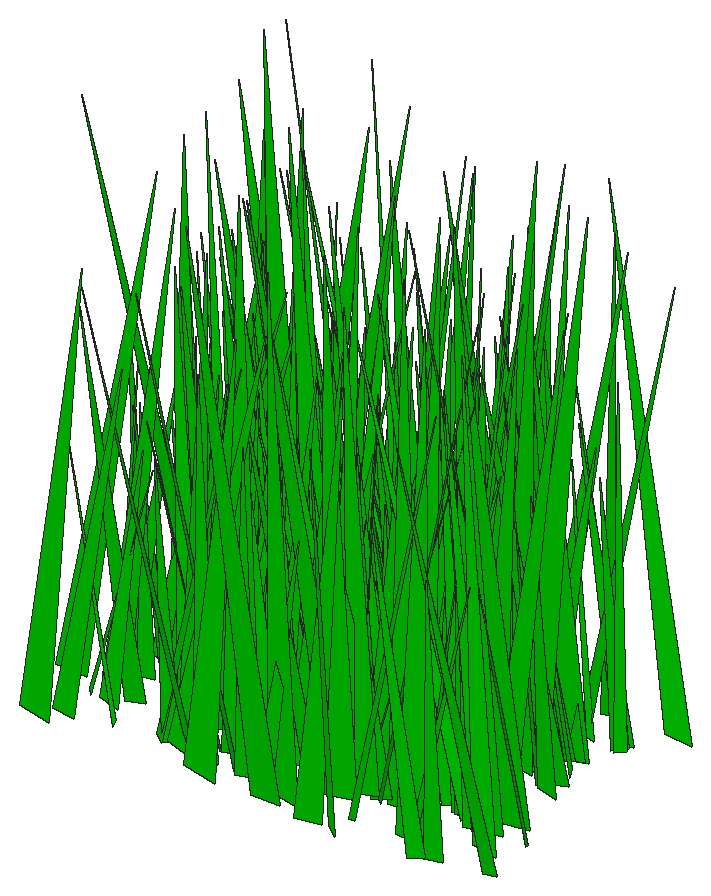
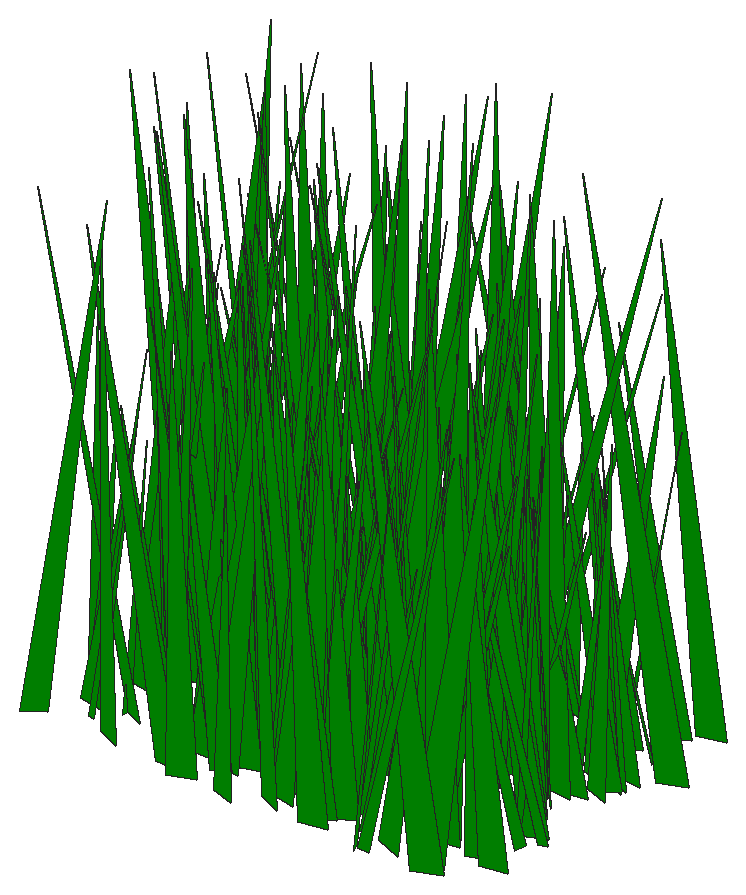
# SketchUp Ruby script. Lengths in inches.
U = 1.inch
M = Sketchup.active_model
def pt(a) = Geom::Point3d.new(a.map { |v| v * U })
def face(e, loops, mat)
  f = e.add_face(loops[0].map { |a| pt(a) })
  loops[1..].each { |l| e.add_face(l.map { |a| pt(a) }).erase! }
  f.material = f.back_material = mat if mat
  f
end
# faces: each face lists its corners as indices into pts; further lists are holes
def faces(e, pts, list, mat = nil) = list.each { |f| face(e, (f[0].is_a?(Array) ? f : [f]).map { |l| l.map { |i| pts[i] } }, mat) }
# xy, xz, yz: faces in a plane at the given z, y or x. An outline is a flat list of corners, or four numbers for a rectangle; further outlines are holes
def ring(l) = l.size == 4 ? [[l[0], l[1]], [l[2], l[1]], [l[2], l[3]], [l[0], l[3]]] : l.each_slice(2).to_a
def flat(e, list, mat, &to3) = list.each { |f| face(e, (f[0].is_a?(Array) ? f : [f]).map { |l| ring(l).map { |u, v| to3.(u, v) } }, mat) }
def xy(e, z, list, mat = nil) = flat(e, list, mat) { |x, y| [x, y, z] }
def xz(e, y, list, mat = nil) = flat(e, list, mat) { |x, z| [x, y, z] }
def yz(e, x, list, mat = nil) = flat(e, list, mat) { |y, z| [x, y, z] }
def lines(e, pts, list) = list.each { |a, b| e.add_line(pt(pts[a]), pt(pts[b])) }
# prism: a flat outline (further loops are holes) pulled along v
def prism(e, loops, v, mat = nil)
  f = face(e, loops, mat); d = Geom::Vector3d.new(v.map { |x| x * U })
  f.pushpull(f.normal.samedirection?(d) ? d.length : -d.length)
end
def box(e, o, s, mat = nil) = prism(e, [[o, [o[0] + s[0], o[1], o[2]], [o[0] + s[0], o[1] + s[1], o[2]], [o[0], o[1] + s[1], o[2]]]], [0, 0, s[2]], mat)
def at(x, y, z, deg = 0) = Geom::Transformation.translation(pt([x, y, z])) * Geom::Transformation.rotation(ORIGIN, Z_AXIS, deg.degrees)
def axes(o, x, y, z) = Geom::Transformation.new([*x, 0, *y, 0, *z, 0, *pt(o).to_a, 1])
def part(name) = M.definitions.add(name)
# library, detail: a bought-in or finely detailed component or shape, given as its bounding box
def library(name, o, s) = part(name).tap { |d| box(d.entities, o, s) }
def detail(e, o, s) = box(e.add_group.entities, o, s)
def put(e, d, t, mat = nil) = e.add_instance(d, t).tap { |i| i.material = mat if mat }
def group(e, t, mat = nil) = e.add_group.tap { |g| g.transformation = t; g.material = mat if mat }.entities
root = M.entities
M.materials.add("[Color G06]").color = [0, 204, 0]
c1 = part("fur_instance\#9")
p = [[0.8125,0,1.79],[0.67,-0.02,1.48],[0,-0.11,0],[0,0.11,0]]
faces(c1.entities,p,[[0,1,2,3]])
put(root,c1,axes([66.86,19.9375,4.28],[1.87865,0.36654,1.99521],[2.70408,-0.30217,0.68954],[-1.17442,-0.10942,4.77928]),"[Color G06]")
put(root,c1,axes([68.1,25.11,4.28],[-2.15525,0.67666,0.22206],[4.83152,0.29674,0.87415],[-0.4748,-0.05194,7.88732]),"[Color G06]")
put(root,c1,axes([67.18,22.58,4.28],[-3.47971,0.08197,1.69373],[0.53126,0.51017,-0.39823],[1.16085,0.01223,5.25931]),"[Color G06]")
put(root,c1,axes([66.52,24.42,4.28],[0.42309,0.57045,0.7628],[4.11466,-0.05401,-0.45808],[0.25485,-0.07503,6.12956]),"[Color G06]")
put(root,c1,axes([66.54,19.3,4.28],[3.07056,-0.08104,1.31793],[-0.44163,-0.44196,-0.8234],[-0.95931,-0.05592,4.59749]),"[Color G06]")
put(root,c1,axes([66.6875,19.39,4.28],[2.45678,0.23622,1.03552],[1.66363,-0.35564,0.50318],[-0.76296,-0.01482,4.43164]),"[Color G06]")
put(root,c1,axes([67.52,19.99,4.28],[-1.9205,-0.283,0.23807],[-1.99672,0.26782,0.59218],[0.39663,-0.02207,4.13384]),"[Color G06]")
put(root,c1,axes([66.43,15.94,4.28],[1.56121,0.60454,1.75227],[4.48997,-0.20626,-0.76122],[0.09967,-0.17771,6.84462]),"[Color G06]")
put(root,c1,axes([68.08,18.0625,4.28],[-1.81069,-0.46934,1.37248],[-3.48469,0.2363,-0.98663],[-0.16937,0.15593,5.62628]),"[Color G06]")
put(root,c1,axes([67.1,24.18,4.28],[-1.84112,0.58038,2.27158],[4.32564,0.28516,-0.53801],[0.96001,-0.17181,6.78063]),"[Color G06]")
put(root,c1,axes([65.73,18.35,4.28],[3.975,-0.58982,0.67635],[-4.2533,-0.55251,0.48784],[-0.07084,0.07718,8.66142]),"[Color G06]")
put(root,c1,axes([67.5,19.25,4.28],[0.83936,0.35374,1.12599],[2.5864,-0.13297,0.49205],[-0.5596,-0.08399,3.96306]),"[Color G06]")
put(root,c1,axes([66.66,19.55,4.28],[2.1428,-0.32761,1.15813],[-2.4734,-0.28656,0.91034],[-0.04931,0.13727,4.66448]),"[Color G06]")
put(root,c1,axes([68.16,24.67,4.28],[-2.63031,-0.31404,1.45688],[-2.40009,0.37075,-0.49867],[0.51157,0.12471,5.15122]),"[Color G06]")
put(root,c1,axes([68.36,16.83,4.28],[-3.11827,0.00052,0.78759],[0.08232,0.43605,0.69466],[0.52051,-0.06582,4.60843]),"[Color G06]")
put(root,c1,axes([67.36,21.62,4.28],[-1.40042,-0.37433,1.56996],[-2.74011,0.22344,0.66016],[0.89517,0.09832,4.47679]),"[Color G06]")
put(root,c1,axes([68.67,23.9,4.28],[-2.32217,-0.30899,0.40673],[-2.22908,0.31788,-0.68694],[-0.12359,0.07246,4.74777]),"[Color G06]")
put(root,c1,axes([67.42,21.06,4.28],[2.68454,-0.01038,1.27198],[0.07883,-0.38667,-0.73394],[-0.85066,-0.06857,3.94611]),"[Color G06]")
put(root,c1,axes([68.76,20.36,4.28],[-2.53339,0.15401,0.39707],[1.13348,0.3487,0.61732],[0.07498,-0.06768,4.08411]),"[Color G06]")
put(root,c1,axes([67.14,20.26,4.28],[1.41484,0.35356,0.45263],[2.55149,-0.19384,-0.42139],[0.10067,-0.05597,4.31898]),"[Color G06]")
put(root,c1,axes([66.32,22.73,4.28],[3.40849,0.26284,0.17789],[1.88535,-0.4715,-0.66404],[0.11163,-0.06222,5.7833]),"[Color G06]")
put(root,c1,axes([70,19.12,4.28],[-5.22641,-0.46331,0.41706],[-3.33362,0.72473,-0.82927],[-0.06343,0.08615,9.21882]),"[Color G06]")
put(root,c1,axes([66.74,22.54,4.28],[2.15826,-0.53872,0.51034],[-3.86774,-0.29494,0.77205],[0.28691,0.07652,6.56871]),"[Color G06]")
put(root,c1,axes([66.82,17.78,4.28],[2.69775,0.05613,0.15937],[0.4148,-0.37075,-0.68549],[-0.03623,-0.06547,4.01857]),"[Color G06]")
put(root,c1,axes([68.17,20.68,4.28],[0.33333,0.50099,1.6784],[3.73976,-0.06195,0.46517],[-0.42793,-0.15115,5.37257]),"[Color G06]")
put(root,c1,axes([67.84,20.44,4.28],[2.61459,-0.6557,1.97081],[-4.76436,-0.38828,-0.72114],[-1.07242,0.12639,8.00869]),"[Color G06]")
put(root,c1,axes([67.875,20.76,4.28],[3.06982,-0.09826,1.8059],[-0.52492,-0.45759,-0.86705],[-1.29654,-0.0474,4.62685]),"[Color G06]")
put(root,c1,axes([66.8,18.875,4.28],[4.09215,-0.51417,0.31047],[-3.65099,-0.56974,-0.89852],[-0.55613,-0.04305,8.18341]),"[Color G06]")
put(root,c1,axes([69.1875,23.38,4.28],[-3.00443,-0.33013,0.34527],[-2.37868,0.41728,-0.40146],[0.01445,0.04936,5.70282]),"[Color G06]")
put(root,c1,axes([68.5,22.24,4.28],[0.12511,0.4386,1.50938],[3.24988,-0.04162,0.78767],[-0.59262,-0.13566,4.63821]),"[Color G06]")
put(root,c1,axes([66.98,16.45,4.28],[2.6605,-0.3964,0.77865],[-2.88966,-0.36648,0.62248],[-0.04716,0.09278,5.7857]),"[Color G06]")
put(root,c1,axes([67.58,17.58,4.28],[0.01908,0.3952,0.29774],[2.79688,0.00227,-0.74606],[0.49908,-0.02781,4.16959]),"[Color G06]")
put(root,c1,axes([67.33,21.74,4.28],[2.2581,-0.40529,1.12701],[-2.99728,-0.31212,0.52087],[-0.17964,0.1131,5.47612]),"[Color G06]")
put(root,c1,axes([66.68,23.17,4.28],[3.54165,-0.16499,0.34756],[-1.2057,-0.48604,0.93878],[-0.018,0.09337,5.50131]),"[Color G06]")
put(root,c1,axes([69.64,25.65,4.28],[-4.18506,0.16157,0.59083],[1.18763,0.58346,0.46238],[0.29713,-0.05642,6.47367]),"[Color G06]")
put(root,c1,axes([67.75,21.26,4.28],[2.76117,0.06081,1.0314],[0.34689,-0.39465,0.59848],[-0.73896,0.04195,4.13483]),"[Color G06]")
put(root,c1,axes([69.21,25.2,4.28],[2.28754,0.39059,3.57758],[3.06302,-0.41996,0.89228],[-2.04786,-0.19184,5.3309]),"[Color G06]")
put(root,c1,axes([68.81,19.81,4.28],[0.33216,-0.36905,1.20751],[-2.69385,-0.06907,-0.76975],[-0.63266,0.10034,3.91151]),"[Color G06]")
put(root,c1,axes([68.78,23.68,4.28],[1.64627,-0.76449,2.9162],[-5.69845,-0.2691,-0.91794],[-1.17939,0.23306,8.50584]),"[Color G06]")
put(root,c1,axes([68.36,24.14,4.28],[-0.90357,-0.68837,2.42229],[-5.14418,0.15076,0.63516],[0.73005,0.2103,7.47357]),"[Color G06]")
put(root,c1,axes([69.47,21.03,4.28],[-3.7436,0.26959,1.66858],[2.08086,0.53147,0.56415],[0.80878,-0.11953,6.27184]),"[Color G06]")
put(root,c1,axes([69.19,20.0625,4.28],[0.16372,-0.57583,0.88536],[-4.12958,-0.03409,-0.84112],[-0.59134,0.07863,6.11904]),"[Color G06]")
put(root,c1,axes([69.25,20.49,4.28],[-4.87639,0.34442,2.38343],[2.40871,0.71498,-0.86054],[1.68574,-0.02531,8.12422]),"[Color G06]")
put(root,c1,axes([69.51,23.16,4.28],[0.01728,0.39517,1.39572],[2.89289,-0.03411,1.02939],[-0.7307,-0.1257,4.10846]),"[Color G06]")
put(root,c1,axes([67.69,25.59,4.28],[2.37057,-0.64778,0.92581],[-4.68012,-0.32216,0.87413],[0.24483,0.11379,7.74547]),"[Color G06]")
put(root,c1,axes([70.09,22.11,4.28],[-2.03665,-0.69248,0.21969],[-4.95861,0.28196,-0.58576],[-0.30712,0.03966,8.00048]),"[Color G06]")
put(root,c1,axes([69.45,20.67,4.28],[-0.23865,0.37319,1.09593],[2.74489,0.0167,0.68194],[-0.40691,-0.10623,3.95739]),"[Color G06]")
put(root,c1,axes([70.99,16.75,4.28],[-4.49676,-0.17942,0.26218],[-1.29851,0.62071,-0.95326],[-0.0085,0.09224,6.92513]),"[Color G06]")
put(root,c1,axes([68.88,21.76,4.28],[2.31214,0.17246,1.55813],[1.49477,-0.32472,-0.82607],[-0.61809,-0.14016,3.8309]),"[Color G06]")
put(root,c1,axes([69.52,23.7,4.28],[-1.56475,-0.35583,1.99839],[-2.84891,0.22263,-0.42902],[0.42773,0.18113,4.45309]),"[Color G06]")
put(root,c1,axes([69.87,25.6875,4.28],[-3.56069,0.01834,1.41738],[0.0277,0.51104,-0.60432],[0.95703,0.05346,5.29094]),"[Color G06]")
put(root,c1,axes([70.14,24.99,4.28],[-2.67002,0.12698,0.6552],[0.96677,0.37124,0.53513],[0.2946,-0.0674,4.18215]),"[Color G06]")
put(root,c1,axes([68.8,19.33,4.28],[2.11124,0.33037,1.52609],[2.57017,-0.28527,-0.84817],[-0.2233,-0.1599,4.6664]),"[Color G06]")
put(root,c1,axes([70.77,24.28,4.28],[-6.01659,-0.01708,1.91793],[-0.04628,0.85646,0.5517],[1.28826,-0.04899,8.97717]),"[Color G06]")
put(root,c1,axes([69.46,24.11,4.28],[3.88439,0.18749,2.22279],[1.24854,-0.58,0.74638],[-1.56873,0.00265,6.09796]),"[Color G06]")
put(root,c1,axes([70.89,20.8,4.28],[1.76802,-0.46536,3.87408],[-3.79882,-0.34664,-0.91072],[-1.85066,0.26697,5.57049]),"[Color G06]")
put(root,c1,axes([69.9375,22.14,4.28],[-2.30921,0.36852,1.8808],[2.72165,0.35258,-0.47168],[1.07715,-0.10084,5.22392]),"[Color G06]")
put(root,c1,axes([70.13,16.98,4.28],[1.25924,-0.38577,0.58888],[-2.69186,-0.18364,-0.96168],[-0.75007,0.01139,4.43995]),"[Color G06]")
put(root,c1,axes([69.6875,18.43,4.28],[2.63574,0.33516,0.9538],[2.34226,-0.37815,0.80643],[-0.83546,-0.00279,5.26991]),"[Color G06]")
put(root,c1,axes([70.56,17.34,4.28],[-2.39176,0.593,0.72625],[4.24328,0.33868,-0.55196],[0.56101,-0.03352,7.2711]),"[Color G06]")
put(root,c1,axes([71.41,17.43,4.28],[-3.23318,-0.07626,0.20624],[-0.5568,0.44941,-0.40903],[0.0899,0.04086,4.88376]),"[Color G06]")
put(root,c1,axes([70.07,22.83,4.28],[3.08996,-0.12092,1.88491],[-1.10884,-0.44997,0.74435],[-1.05497,0.11878,4.73848]),"[Color G06]")
put(root,c1,axes([71.2,22.44,4.28],[-1.9391,-0.26111,1.2844],[-2.05387,0.25798,-0.90149],[0.16274,0.14464,3.92666]),"[Color G06]")
put(root,c1,axes([72.3125,16.91,4.28],[-4.63411,-0.11914,0.54552],[-0.90008,0.63988,-1.0263],[0.23024,0.10358,6.96756]),"[Color G06]")
put(root,c1,axes([72.5625,23.87,4.28],[-5.03737,0.15992,0.47896],[1.16716,0.7016,0.50985],[0.23592,-0.05637,7.70452]),"[Color G06]")
put(root,c1,axes([70.64,17.21,4.28],[1.92034,0.64349,1.46988],[4.66024,-0.28183,0.57361],[-0.73787,-0.10529,7.44824]),"[Color G06]")
put(root,c1,axes([71.47,20.19,4.28],[-3.19334,0.26439,1.99081],[2.16495,0.45316,0.84359],[0.82592,-0.16563,5.48606]),"[Color G06]")
put(root,c1,axes([71.6,18.84,4.28],[-3.18635,0.38671,0.67327],[2.69516,0.44754,-1.0376],[0.79354,0.03276,6.22746]),"[Color G06]")
put(root,c1,axes([71.7,24.47,4.28],[2.18816,0.37389,2.89627],[2.82521,-0.37976,0.86384],[-1.72125,-0.14801,5.09981]),"[Color G06]")
put(root,c1,axes([70.85,24.09,4.28],[-0.32978,0.44304,1.07825],[3.23647,0.05616,-0.43984],[0.37426,-0.09529,4.75371]),"[Color G06]")
put(root,c1,axes([71.62,24.69,4.28],[-5.44694,0.14293,2.6999],[0.9286,0.8,-0.68034],[1.85785,0.01918,8.25575]),"[Color G06]")
put(root,c1,axes([70.64,18.29,4.28],[2.65428,-0.46035,0.81882],[-3.27632,-0.37734,-0.64678],[-0.68156,0.0211,6.29791]),"[Color G06]")
put(root,c1,axes([69.76,16.96,4.28],[4.07276,0.1691,0.72699],[1.2606,-0.56695,-0.62595],[-0.34363,-0.0756,6.32022]),"[Color G06]")
put(root,c1,axes([71.48,16.72,4.28],[0.89866,0.51945,1.33537],[3.77379,-0.14203,0.67396],[-0.6582,-0.10513,5.68738]),"[Color G06]")
put(root,c1,axes([70.92,24.74,4.28],[-2.03427,0.47242,2.51983],[3.53808,0.33213,-0.77265],[1.34233,-0.15948,5.85528]),"[Color G06]")
put(root,c1,axes([71.08,19.01,4.28],[-1.9152,0.36614,2.16956],[2.68071,0.31667,-0.85322],[1.34728,-0.10962,4.78176]),"[Color G06]")
put(root,c1,axes([71.48,19.53,4.28],[2.66418,0.13711,1.46624],[0.87126,-0.39543,0.71164],[-1.08175,0.01921,4.18426]),"[Color G06]")
put(root,c1,axes([71.09,18.5,4.28],[2.67934,-0.3919,0.38989],[-2.74937,-0.37373,-0.94945],[-0.63841,-0.03529,5.72518]),"[Color G06]")
put(root,c1,axes([70.22,23.08,4.28],[4.92283,0.46681,1.55066],[3.44128,-0.69107,-0.50511],[-0.66366,-0.12078,8.88315]),"[Color G06]")
put(root,c1,axes([71.08,18.49,4.28],[-0.01067,0.39008,0.75182],[2.75792,0.01838,-1.0079],[0.68705,-0.06771,4.05756]),"[Color G06]")
put(root,c1,axes([72.54,17.95,4.28],[-3.20854,0.5435,2.05319],[4.10111,0.44865,0.67282],[0.50943,-0.18866,7.51511]),"[Color G06]")
put(root,c1,axes([73.02,20.01,4.28],[-3.27762,0.0696,0.09378],[0.5027,0.45527,0.43295],[0.01818,-0.04125,4.93616]),"[Color G06]")
put(root,c1,axes([72.61,23.23,4.28],[-3.36746,-0.11854,0.93472],[-0.91893,0.47275,-0.50766],[0.51901,0.06791,5.16592]),"[Color G06]")
put(root,c1,axes([71.39,25.47,4.28],[0.0515,0.59852,1.18292],[4.35167,0.00142,-0.50587],[0.33469,-0.11059,6.39544]),"[Color G06]")
put(root,c1,axes([71.39,18.27,4.28],[0.1555,-0.38375,1.24845],[-2.85704,-0.00724,0.53918],[0.32964,0.11826,4.08421]),"[Color G06]")
put(root,c1,axes([70.56,16.81,4.28],[2.68875,0.54608,0.55936],[3.92681,-0.36876,-0.80773],[0.23645,-0.08553,7.05353]),"[Color G06]")
put(root,c1,axes([72.42,24.54,4.28],[2.08905,-0.57183,2.84194],[-4.26391,-0.34625,-1.00203],[-1.50031,0.18783,6.80495]),"[Color G06]")
put(root,c1,axes([71.76,19.93,4.28],[-2.5059,-0.08559,2.17745],[-0.46067,0.40376,0.63892],[1.51231,-0.01883,3.80266]),"[Color G06]")
put(root,c1,axes([71.65,22.36,4.28],[0.04403,-0.55707,0.45266],[-3.97735,-0.001,0.72254],[0.48148,0.04267,5.92718]),"[Color G06]")
put(root,c1,axes([71.96,17.59,4.28],[2.49858,-0.7621,1.22476],[-5.44507,-0.36092,-0.98619],[-0.94432,0.06469,8.92705]),"[Color G06]")
put(root,c1,axes([71.375,25.08,4.28],[2.08427,-0.50925,1.70734],[-3.82608,-0.27986,0.84419],[-0.05277,0.17755,6.22752]),"[Color G06]")
put(root,c1,axes([72.76,24.9375,4.28],[-0.44557,0.41686,0.30084],[2.96924,0.05764,0.64874],[-0.4009,-0.03642,4.47043]),"[Color G06]")
put(root,c1,axes([72.89,20,4.28],[2.34818,-0.68971,3.6819],[-5.24588,-0.39553,-1.038],[-1.73598,0.26228,8.11702]),"[Color G06]")
put(root,c1,axes([71.6,19.62,4.28],[1.93818,-0.4421,1.09106],[-3.25174,-0.26704,0.473],[-0.1042,0.11,5.53358]),"[Color G06]")
put(root,c1,axes([71.77,16.1,4.28],[0.44845,-0.59229,2.57221],[-4.55599,-0.03154,0.93997],[0.49558,0.24599,6.31381]),"[Color G06]")
put(root,c1,axes([72.95,19.9,4.28],[-4.47212,0.45643,2.42543],[3.3283,0.6565,-0.48377],[1.50651,-0.09547,8.26875]),"[Color G06]")
put(root,c1,axes([73.09,24.83,4.28],[-3.85958,0.09549,1.77507],[0.79917,0.55874,0.4286],[1.11393,-0.07,5.84281]),"[Color G06]")
put(root,c1,axes([74.125,22.51,4.28],[-4.09834,-0.08446,0.1041],[-0.59159,0.56687,0.80859],[0.14742,-0.07323,6.13878]),"[Color G06]")
put(root,c1,axes([72.22,20.39,4.28],[2.5598,0.08888,0.95436],[0.55163,-0.36615,0.61199],[-0.71391,0.03576,3.89483]),"[Color G06]")
put(root,c1,axes([72.79,16.75,4.28],[0.83062,0.44946,0.92704],[3.2366,-0.127,0.59543],[-0.5461,-0.06905,4.93894]),"[Color G06]")
put(root,c1,axes([74.5625,18.74,4.28],[-3.75514,0.60555,0.30301],[4.33004,0.51767,1.02411],[-0.38697,-0.08377,8.51899]),"[Color G06]")
put(root,c1,axes([72.64,23.35,4.28],[-1.03716,-0.47927,0.64226],[-3.42165,0.15149,0.64364],[0.53848,0.03948,5.3269]),"[Color G06]")
put(root,c1,axes([73.96,16.11,4.28],[-3.38072,-0.6515,1.18354],[-4.7345,0.47012,-0.48048],[0.20061,0.11585,8.60575]),"[Color G06]")
put(root,c1,axes([73.28,24.41,4.28],[0.14572,0.47172,1.353],[3.44856,-0.04129,0.82385],[-0.6085,-0.12101,4.99302]),"[Color G06]")
put(root,c1,axes([73.45,17.98,4.28],[-4.82019,0.18669,2.80146],[1.64531,0.70331,0.93941],[1.6121,-0.15958,7.4176]),"[Color G06]")
put(root,c1,axes([72.91,25.28,4.28],[3.98745,0.36913,2.2275],[2.62685,-0.59121,0.75083],[-1.52584,-0.05318,7.1137]),"[Color G06]")
put(root,c1,axes([74.33,17.61,4.28],[-2.66251,-0.38327,0.56727],[-2.77455,0.36742,-0.57227],[-0.0136,0.07516,5.6905]),"[Color G06]")
put(root,c1,axes([72.65,24.36,4.28],[-3.51567,0.38725,3.93085],[2.92412,0.59324,-0.87178],[2.46556,-0.15139,6.63897]),"[Color G06]")
put(root,c1,axes([74.94,17.91,4.28],[-4.13497,-0.64011,0.27453],[-4.57391,0.57684,0.6177],[0.42988,-0.0196,9.21303]),"[Color G06]")
put(root,c1,axes([74.85,19.2,4.28],[-3.04007,-0.00929,0.08099],[-0.07298,0.42055,-0.57577],[0.0453,0.05388,4.50807]),"[Color G06]")
put(root,c1,axes([73.07,20.16,4.28],[1.0003,0.60058,0.32674],[4.30713,-0.13758,-0.40367],[0.21404,-0.03817,6.59597]),"[Color G06]")
put(root,c1,axes([72.99,18.82,4.28],[2.43837,-0.47266,1.51337],[-3.52645,-0.33836,0.55203],[-0.28047,0.14512,6.21614]),"[Color G06]")
put(root,c1,axes([72.95,23.84,4.28],[2.42602,0.30934,1.01152],[2.3127,-0.33296,-0.693],[-0.17501,-0.11177,4.86408]),"[Color G06]")
put(root,c1,axes([73.51,23.26,4.28],[2.38039,-0.30927,0.62713],[-2.12557,-0.33575,-0.99807],[-0.75946,-0.02966,4.75901]),"[Color G06]")
put(root,c1,axes([72.1,20.48,4.28],[5.1034,0.13112,0.77105],[0.98866,-0.71072,-0.73318],[-0.41576,-0.08058,7.72107]),"[Color G06]")
put(root,c1,axes([74.04,25.71,4.28],[1.22243,0.36432,1.21108],[2.64683,-0.18878,0.55616],[-0.69063,-0.07865,4.27508]),"[Color G06]")
put(root,c1,axes([73.09,20.41,4.28],[4.77794,-0.34193,2.51952],[-2.71041,-0.68361,0.8239],[-1.22807,0.17845,7.98408]),"[Color G06]")
put(root,c1,axes([74.25,16.46,4.28],[-2.29012,-0.66362,1.93208],[-4.85109,0.33889,0.52704],[0.88644,0.14012,7.87571]),"[Color G06]")
put(root,c1,axes([73.14,20.8,4.28],[1.53952,0.3889,0.27764],[2.75365,-0.20595,-0.96734],[0.4797,-0.0659,4.66187]),"[Color G06]")
put(root,c1,axes([73.64,16.36,4.28],[0.15856,0.36146,1.34529],[2.68142,0.00628,-0.89975],[0.5825,-0.1273,3.77564]),"[Color G06]")
put(root,c1,axes([74.64,22.86,4.28],[-0.15453,-0.60751,0.79266],[-4.37376,0.0152,-0.56629],[-0.36272,0.07552,6.49072]),"[Color G06]")
put(root,c1,axes([74.88,24.59,4.28],[-1.3305,-0.56696,0.95717],[-4.11502,0.18121,-0.44658],[-0.08845,0.09777,6.37818]),"[Color G06]")
put(root,c1,axes([73.92,23.125,4.28],[-0.01043,-0.53939,1.54118],[-3.9819,0.01621,0.59164],[0.41245,0.14288,5.75084]),"[Color G06]")
put(root,c1,axes([75.22,19.31,4.28],[-3.62133,0.55392,2.01147],[4.14686,0.50999,0.54329],[0.62771,-0.17358,8.0153]),"[Color G06]")
put(root,c1,axes([74.83,20.85,4.28],[-0.73506,-0.45535,0.90726],[-3.31658,0.09598,-0.46869],[-0.17821,0.09198,4.98053]),"[Color G06]")
put(root,c1,axes([74.22,19.78,4.28],[3.45704,0.03016,1.8901],[0.3316,-0.51062,-0.41874],[-1.23941,-0.05249,5.15993]),"[Color G06]")
put(root,c1,axes([73.93,18.95,4.28],[2.64155,-0.10718,0.52359],[-0.67976,-0.36495,-0.92095],[-0.50137,-0.06987,4.00725]),"[Color G06]")
put(root,c1,axes([74.21,22.07,4.28],[2.32397,-0.26492,0.35706],[-1.81842,-0.32177,-0.98704],[-0.59974,-0.05096,4.37631]),"[Color G06]")
put(root,c1,axes([74.63,18.97,4.28],[2.11562,0.26123,1.46079],[1.90426,-0.3193,0.39892],[-0.91571,-0.06047,4.20452]),"[Color G06]")
put(root,c1,axes([73.55,22.09,4.28],[5.72613,-0.10854,2.10438],[-0.87942,-0.81899,0.49278],[-1.3472,0.07329,8.62276]),"[Color G06]")
put(root,c1,axes([75.71,24.42,4.28],[-3.28874,-0.6312,0.25941],[-4.51722,0.45922,0.43468],[0.33729,-0.0043,8.35093]),"[Color G06]")
put(root,c1,axes([75.07,22.66,4.28],[0.05868,-0.45361,1.16943],[-3.32151,-0.021,-0.56336],[-0.40164,0.10738,4.82979]),"[Color G06]")
put(root,c1,axes([74.82,20.08,4.28],[1.59256,-0.33392,0.11223],[-2.31659,-0.21784,-1.02366],[-0.61089,-0.04444,4.17445]),"[Color G06]")
put(root,c1,axes([74.73,23.58,4.28],[3.96852,0.14607,2.60004],[1.33557,-0.5889,-0.75302],[-1.52967,-0.13522,6.08799]),"[Color G06]")
put(root,c1,axes([75.1875,18.93,4.28],[-1.60635,-0.45647,0.89354],[-3.28248,0.23256,0.4662],[0.54618,0.05515,5.42977]),"[Color G06]")
put(root,c1,axes([76.21,19.56,4.28],[-2.54648,0.22504,0.37084],[1.62695,0.34431,0.95346],[-0.13781,-0.0935,4.40379]),"[Color G06]")
put(root,c1,axes([74.43,24.27,4.28],[2.30861,-0.56144,1.86697],[-4.20491,-0.32079,0.53286],[-0.29923,0.17628,6.916]),"[Color G06]")
put(root,c1,axes([75.36,17.42,4.28],[1.76853,-0.69807,2.35607],[-5.15587,-0.27444,-0.69583],[-0.98101,0.18391,7.90448]),"[Color G06]")
put(root,c1,axes([75.5,23.01,4.28],[-1.71907,0.42142,0.28388],[2.98576,0.24098,-0.70607],[0.50429,0.00981,5.14815]),"[Color G06]")
put(root,c1,axes([75.04,17.75,4.28],[-3.57411,0.55685,3.14119],[4.08288,0.55827,-0.9918],[1.92201,-0.15041,7.94808]),"[Color G06]")
put(root,c1,axes([75.4375,25.6,4.28],[-1.35298,0.6098,0.14784],[4.33758,0.18891,-0.83744],[0.56443,0.01002,6.79004]),"[Color G06]")
put(root,c1,axes([75.9,24.125,4.28],[-0.49053,0.49413,1.28889],[3.63769,0.05764,0.55405],[-0.26011,-0.12577,5.31781]),"[Color G06]")
put(root,c1,axes([75.72,17.94,4.28],[1.74822,-0.62493,2.01501],[-4.56579,-0.2718,-0.83507],[-1.02725,0.14456,7.14088]),"[Color G06]")
put(root,c1,axes([74.84,24.77,4.28],[1.12479,-0.42454,0.34104],[-3.04222,-0.153,0.5329],[0.25668,0.04694,4.82146]),"[Color G06]")
put(root,c1,axes([74.93,21.45,4.28],[1.95762,-0.35544,1.20971],[-2.66575,-0.27058,0.50329],[-0.21488,0.11852,4.77706]),"[Color G06]")
put(root,c1,axes([76.28,18.02,4.28],[-0.49801,-0.45175,1.4283],[-3.32828,0.04269,-1.04119],[-0.57535,0.14408,4.7868]),"[Color G06]")
put(root,c1,axes([75.74,19.81,4.28],[-2.40754,-0.24451,1.38579],[-1.73571,0.35812,0.5229],[0.96003,0.03429,4.42063]),"[Color G06]")
put(root,c1,axes([75.6,23.48,4.28],[-2.32222,0.50185,2.26997],[3.69756,0.36186,-0.74078],[1.25982,-0.137,6.35842]),"[Color G06]")
put(root,c1,axes([76.01,19.76,4.28],[-1.3295,-0.46342,0.74573],[-3.33211,0.1915,0.40129],[0.43651,0.05038,5.3346]),"[Color G06]")
put(root,c1,axes([75.5,15.9375,4.28],[1.94351,0.61242,0.16127],[4.36922,-0.27117,0.6773],[-0.45798,0.01188,7.14589]),"[Color G06]")
put(root,c1,axes([75.29,19.22,4.28],[0.53155,-0.62868,1.95305],[-4.67424,-0.05407,0.8422],[0.43053,0.18914,6.73243]),"[Color G06]")
put(root,c1,axes([76.17,24.91,4.28],[3.40234,0.31823,3.65359],[2.84004,-0.53172,-0.58742],[-1.76585,-0.24202,6.09478]),"[Color G06]")
put(root,c1,axes([76.33,15.9,4.28],[-3.41465,-0.21549,1.6466],[-1.43725,0.50014,0.86129],[1.23944,-0.01372,5.53514]),"[Color G06]")
put(root,c1,axes([74.92,20.83,4.28],[3.37448,-0.3812,0.70367],[-2.77112,-0.46794,0.56371],[-0.12564,0.08228,6.46619]),"[Color G06]")
put(root,c1,axes([75.93,22.18,4.28],[0.3588,-0.5941,0.61938],[-4.27348,-0.04638,0.41904],[0.24599,0.06076,6.37634]),"[Color G06]")
put(root,c1,axes([75.3,24.52,4.28],[4.20367,-0.03528,1.06715],[-0.16518,-0.59061,-0.78926],[-0.73927,-0.06862,6.24438]),"[Color G06]")
put(root,c1,axes([75.5625,23.58,4.28],[1.42316,-0.79981,1.58928],[-5.82538,-0.18686,0.84986],[0.30586,0.16265,8.79134]),"[Color G06]")
put(root,c1,axes([75.05,23.97,4.28],[4.90177,-0.48381,0.58116],[-3.43131,-0.68486,-0.84697],[-0.64405,-0.03345,8.93547]),"[Color G06]")
put(root,c1,axes([75.72,21,4.28],[4.71467,0.06861,1.91609],[0.64269,-0.6752,-0.75506],[-1.21352,-0.09103,7.04434]),"[Color G06]")
put(root,c1,axes([77.91,18.98,4.28],[-3.88706,0.42449,1.36908],[3.16269,0.53678,0.93898],[0.32136,-0.14827,7.31903]),"[Color G06]")
put(root,c1,axes([76.36,19.59,4.28],[-3.59873,0.41951,4.54753],[3.74492,0.57698,0.50545],[2.06982,-0.31455,6.99215]),"[Color G06]")
put(root,c1,axes([78.73,18.57,4.28],[-4.70649,0.23242,0.05592],[1.66582,0.65498,0.45709],[-0.0669,-0.04194,7.44825]),"[Color G06]")
put(root,c1,axes([75.66,21.43,4.28],[4.05511,0.38996,0.65923],[2.77897,-0.5688,0.46713],[-0.54052,0.00117,7.34724]),"[Color G06]")
put(root,c1,axes([77.64,23.54,4.28],[-2.76992,0.3822,0.3991],[2.72409,0.38802,-0.4541],[0.40344,0.00408,5.80623]),"[Color G06]")
put(root,c1,axes([77.0625,18,4.28],[1.18021,0.69682,2.29982],[5.18835,-0.18333,0.43338],[-0.64774,-0.19879,7.66171]),"[Color G06]")
put(root,c1,axes([75.33,18.57,4.28],[4.56317,0.0628,0.11517],[0.44063,-0.63338,0.67896],[-0.12094,0.062,6.81942]),"[Color G06]")
put(root,c1,axes([76.66,24.08,4.28],[4.45429,-0.38562,2.02219],[-2.76097,-0.64717,-0.59203],[-1.362,0.05077,7.81351]),"[Color G06]")
put(root,c1,axes([76.3,22.46,4.28],[5.56447,0.35267,1.64159],[2.45006,-0.79066,0.96175],[-1.2649,0.01998,9.08445]),"[Color G06]")
put(root,c1,axes([76.03,25.37,4.28],[4.20271,-0.4361,0.17603],[-3.11555,-0.5856,-0.50608],[-0.29649,-0.02811,7.81318]),"[Color G06]")
put(root,c1,axes([76.37,19.4,4.28],[2.61625,0.35712,0.34103],[2.55257,-0.35532,-0.99924],[0.30827,-0.08864,5.3797]),"[Color G06]")
put(root,c1,axes([76.35,16.7,4.28],[4.57437,-0.03562,0.84842],[-0.29779,-0.64074,0.49592],[-0.54665,0.05095,6.8294]),"[Color G06]")
put(root,c1,axes([77.86,21.32,4.28],[-2.48839,0.24398,1.5767],[1.73916,0.37461,-0.52777],[1.07212,-0.04141,4.51564]),"[Color G06]")
put(root,c1,axes([78.84,22.64,4.28],[-2.73148,-0.23271,0.8254],[-1.75382,0.37042,-0.96729],[0.11912,0.11747,4.68524]),"[Color G06]")
put(root,c1,axes([76.33,17.88,4.28],[5.39592,0.05224,1.01834],[0.29087,-0.7534,0.99716],[-0.72111,0.08702,8.02227]),"[Color G06]")
put(root,c1,axes([77.26,23.87,4.28],[0.42983,0.40442,1.27891],[2.96963,-0.03374,-1.00381],[0.56998,-0.1292,4.26544]),"[Color G06]")
put(root,c1,axes([77.87,23.21,4.28],[-2.9741,-0.0563,2.2633],[-0.63177,0.4576,-0.54671],[1.43427,0.08481,4.45234]),"[Color G06]")
put(root,c1,axes([78.34,18.76,4.28],[-3.2756,0.31968,2.31275],[2.54022,0.48002,0.4145],[1.09421,-0.1574,5.9611]),"[Color G06]")
put(root,c1,axes([78.06,25.18,4.28],[3.81515,0.36125,2.48742],[2.58786,-0.57642,0.75055],[-1.6686,-0.06801,6.85137]),"[Color G06]")
put(root,c1,axes([78.9,16.18,4.28],[-2.22535,0.33327,1.05822],[2.48876,0.30444,0.67672],[0.13876,-0.11559,4.83351]),"[Color G06]")
put(root,c1,axes([79.25,22.17,4.28],[-4.49658,-0.04815,1.15535],[-0.24136,0.6313,0.92402],[0.81151,-0.07904,6.67661]),"[Color G06]")
put(root,c1,axes([78.51,23.89,4.28],[-2.57213,0.11979,1.01712],[0.78559,0.37033,-0.57284],[0.76419,0.0225,4.01231]),"[Color G06]")
put(root,c1,axes([79.04,24.625,4.28],[-3.74738,0.02989,1.1622],[0.2911,0.53069,0.52869],[0.75226,-0.05646,5.58492]),"[Color G06]")
put(root,c1,axes([78.83,22.71,4.28],[-0.71146,-0.57833,1.56638],[-4.26398,0.084,-0.76324],[-0.34281,0.15538,6.2426]),"[Color G06]")
put(root,c1,axes([79.35,21.44,4.28],[-1.46718,-0.56789,0.24395],[-4.0359,0.19905,-0.9894],[-0.56858,0.05247,6.39348]),"[Color G06]")
put(root,c1,axes([77.82,21.58,4.28],[-0.48994,-0.7576,1.82571],[-5.51964,0.0887,0.91942],[0.73688,0.16067,8.10092]),"[Color G06]")
put(root,c1,axes([78.95,21.15,4.28],[-3.63212,-0.10343,1.65999],[-0.88339,0.52262,-0.57702],[1.00167,0.08588,5.51037]),"[Color G06]")
put(root,c1,axes([78.59,18.65,4.28],[3.49328,0.49629,3.07989],[3.70969,-0.54301,0.65292],[-1.77529,-0.15812,7.42474]),"[Color G06]")
put(root,c1,axes([78.32,16.79,4.28],[-1.5005,0.65628,2.54496],[4.93593,0.23507,-0.46281],[0.82829,-0.21191,7.36834]),"[Color G06]")
put(root,c1,axes([78.93,22.72,4.28],[0.41125,-0.61022,1.03327],[-4.38891,-0.06933,-0.80142],[-0.60463,0.08818,6.52013]),"[Color G06]")
put(root,c1,axes([78.0625,20.35,4.28],[-0.73253,-0.60902,2.06609],[-4.49296,0.13361,0.96587],[0.8939,0.17246,6.54782]),"[Color G06]")
put(root,c1,axes([77.63,19.26,4.28],[5.43479,-0.07218,2.05672],[-0.61964,-0.77883,0.51757],[-1.3333,0.06773,8.14302]),"[Color G06]")
put(root,c1,axes([79.48,24.11,4.28],[-1.85573,0.35531,0.83987],[2.60854,0.25041,0.70503],[-0.06022,-0.10197,4.65807]),"[Color G06]")
put(root,c1,axes([79.33,18.35,4.28],[-3.50579,0.3014,2.15861],[2.42664,0.5007,0.77236],[0.9323,-0.16986,6.1068]),"[Color G06]")
put(root,c1,axes([79.39,18.34,4.28],[-0.83955,0.81715,1.99827],[6.00293,0.10447,0.72594],[-0.30394,-0.19378,8.81785]),"[Color G06]")
put(root,c1,axes([80.77,18.45,4.28],[-6.00693,-0.11984,0.89464],[-0.91486,0.83697,-0.84224],[0.5098,0.08994,9.03002]),"[Color G06]")
put(root,c1,axes([80.34,25.27,4.28],[-4.52932,0.48421,0.45751],[3.4396,0.63217,-0.79522],[0.56607,0.03311,8.4927]),"[Color G06]")
put(root,c1,axes([79.83,19.06,4.28],[-1.81991,-0.68742,1.66118],[-5.05311,0.24575,-0.68392],[-0.05531,0.16743,7.82395]),"[Color G06]")
put(root,c1,axes([78.24,21.68,4.28],[1.50061,0.77959,1.76533],[5.70749,-0.19635,-0.87661],[0.27352,-0.1799,8.60685]),"[Color G06]")
put(root,c1,axes([78.5,16.92,4.28],[2.72255,0.09086,1.07602],[0.79162,-0.38075,-0.78095],[-0.56231,-0.09612,4.11041]),"[Color G06]")
put(root,c1,axes([79.35,16.34,4.28],[0.42966,0.40214,0.74404],[2.89472,-0.06871,0.53232],[-0.43019,-0.06072,4.32508]),"[Color G06]")
put(root,c1,axes([79.46,23.9375,4.28],[1.23035,-0.35197,0.86994],[-2.45552,-0.18709,-0.93779],[-0.82461,0.03196,4.09055]),"[Color G06]")
put(root,c1,axes([78.35,16.68,4.28],[2.73091,0.17554,0.17925],[1.24168,-0.37977,0.46779],[-0.23946,0.0327,4.46992]),"[Color G06]")
put(root,c1,axes([79.45,20.93,4.28],[-1.43314,-0.39895,0.46397],[-2.83652,0.20399,0.57795],[0.48539,0.01416,4.74735]),"[Color G06]")
put(root,c1,axes([78.29,20.59,4.28],[3.45524,-0.49702,1.3632],[-3.66016,-0.48206,0.53277],[-0.37299,0.12626,7.40012]),"[Color G06]")
put(root,c1,axes([80.97,16.65,4.28],[-3.49503,-0.34353,0.40026],[-2.4768,0.48219,-0.76887],[-0.07966,0.08011,6.34441]),"[Color G06]")
put(root,c1,axes([79.57,23.83,4.28],[-3.12534,0.17761,2.50848],[1.5699,0.47555,0.50125],[1.40523,-0.13626,5.01907]),"[Color G06]")
put(root,c1,axes([80.08,17.55,4.28],[-3.7934,0.43521,1.49435],[3.06423,0.54664,-0.91323],[1.16229,-0.02075,7.28476]),"[Color G06]")
put(root,c1,axes([78.22,23.97,4.28],[4.59833,0.3104,0.6254],[2.20516,-0.64369,0.48192],[-0.51685,0.01523,7.6202]),"[Color G06]")
